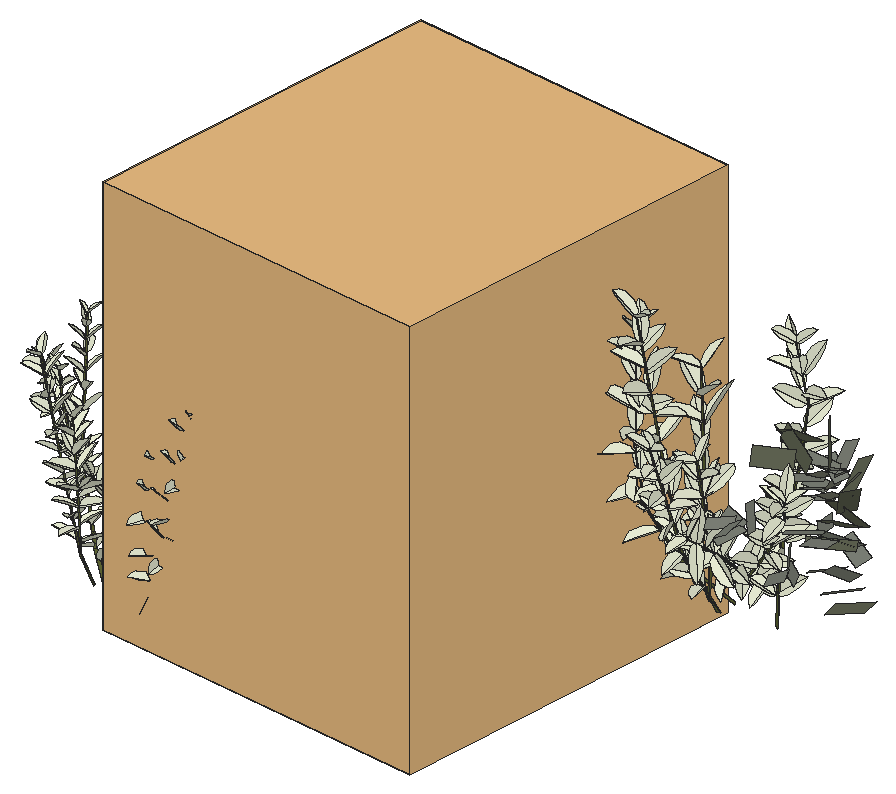
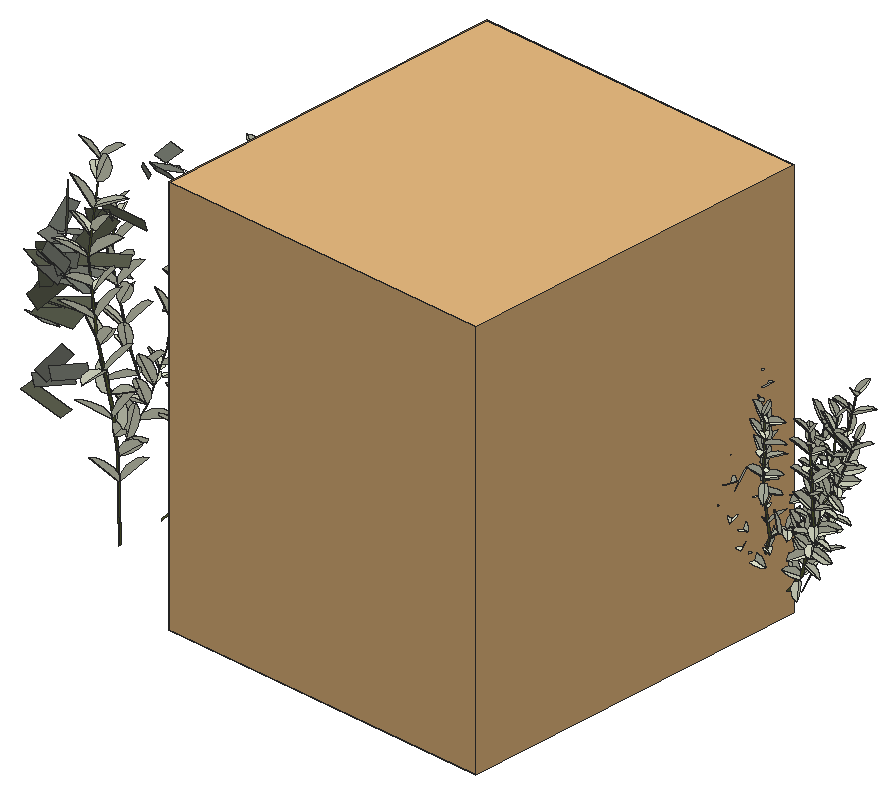
# SketchUp Ruby script. Lengths in inches.
U = 1.inch
M = Sketchup.active_model
def pt(a) = Geom::Point3d.new(a.map { |v| v * U })
def face(e, loops, mat)
  f = e.add_face(loops[0].map { |a| pt(a) })
  loops[1..].each { |l| e.add_face(l.map { |a| pt(a) }).erase! }
  f.material = f.back_material = mat if mat
  f
end
# faces: each face lists its corners as indices into pts; further lists are holes
def faces(e, pts, list, mat = nil) = list.each { |f| face(e, (f[0].is_a?(Array) ? f : [f]).map { |l| l.map { |i| pts[i] } }, mat) }
# xy, xz, yz: faces in a plane at the given z, y or x. An outline is a flat list of corners, or four numbers for a rectangle; further outlines are holes
def ring(l) = l.size == 4 ? [[l[0], l[1]], [l[2], l[1]], [l[2], l[3]], [l[0], l[3]]] : l.each_slice(2).to_a
def flat(e, list, mat, &to3) = list.each { |f| face(e, (f[0].is_a?(Array) ? f : [f]).map { |l| ring(l).map { |u, v| to3.(u, v) } }, mat) }
def xy(e, z, list, mat = nil) = flat(e, list, mat) { |x, y| [x, y, z] }
def xz(e, y, list, mat = nil) = flat(e, list, mat) { |x, z| [x, y, z] }
def yz(e, x, list, mat = nil) = flat(e, list, mat) { |y, z| [x, y, z] }
def lines(e, pts, list) = list.each { |a, b| e.add_line(pt(pts[a]), pt(pts[b])) }
# prism: a flat outline (further loops are holes) pulled along v
def prism(e, loops, v, mat = nil)
  f = face(e, loops, mat); d = Geom::Vector3d.new(v.map { |x| x * U })
  f.pushpull(f.normal.samedirection?(d) ? d.length : -d.length)
end
def box(e, o, s, mat = nil) = prism(e, [[o, [o[0] + s[0], o[1], o[2]], [o[0] + s[0], o[1] + s[1], o[2]], [o[0], o[1] + s[1], o[2]]]], [0, 0, s[2]], mat)
def at(x, y, z, deg = 0) = Geom::Transformation.translation(pt([x, y, z])) * Geom::Transformation.rotation(ORIGIN, Z_AXIS, deg.degrees)
def axes(o, x, y, z) = Geom::Transformation.new([*x, 0, *y, 0, *z, 0, *pt(o).to_a, 1])
def part(name) = M.definitions.add(name)
# library, detail: a bought-in or finely detailed component or shape, given as its bounding box
def library(name, o, s) = part(name).tap { |d| box(d.entities, o, s) }
def detail(e, o, s) = box(e.add_group.entities, o, s)
def put(e, d, t, mat = nil) = e.add_instance(d, t).tap { |i| i.material = mat if mat }
def group(e, t, mat = nil) = e.add_group.tap { |g| g.transformation = t; g.material = mat if mat }.entities
root = M.entities
M.materials.add("0ad16as01f6asdLeafVar1sfd015as60f1as6").color = [231, 235, 211]
M.materials.add("asdfasdf0165f6asdLeafVar1sfd015as60f1as6").color = [231, 235, 211]
M.materials.add("dw_stemssadfasdfa0sdf1s01d6w1").color = [90, 97, 50]
M.materials.add("viburnumblaasdfas0df1w06d").color = [98, 102, 84]
M.materials.add("viburnumbladsadfasdfad0w122").color = [125, 129, 119]
c1 = part("vdw_leaf\#2")
p = [[0,0,0],[-2.77,1.61,2.32],[-4.3125,6.1,4.5],[-3.97,13.49,6.09],[-2.47,18.57,6.3],[-0.2,22.73,5.75],
  [2.54,19.66,6.85],[4.3,15.93,7.09],[5.03,7.6,5.43],[3.32,1.76,2.74]]
faces(c1.entities,p,[[0,1,2,3,4,5],[0,5,6,7,8,9]],"asdfasdf0165f6asdLeafVar1sfd015as60f1as6")
c2 = part("dg_branch_1\#2")
p = [[46.12,1.57,35.62],[46,5.42,35.41],[0.14,1.79,0.05],[0.26,-2.0625,0.27],[74.05,2.99,75.8],[74.11,5.28,75.58],
  [103.46,0.47,94.74],[104.03,2.92,94.84],[81.14,16.92,120.46],[81.2,18.78,120.24],[130.47,-5.6875,130.27],[130.58,-3.66,129.85],
  [80.82,34.4375,191.22],[80.64,35.93,190.9],[148.49,-14.56,203.24],[148.9,-12.8125,203.11],[81.08,37.95,226.93],[81.4,39.1,227.03],
  [157.45,-18.19,250.77],[157.7,-17.01,250.41]]
faces(c2.entities,p,[[0,1,2,3],[4,0,1],[4,1,5],[6,4,5],[6,5,7],[8,4,5],[8,5,9],[10,6,7],
  [10,7,11],[12,8,9],[12,9,13],[14,10,11],[14,11,15],[16,12,13],[16,13,17],[18,14,15],
  [18,15,19]],"dw_stemssadfasdfa0sdf1s01d6w1")
c3 = part("vdw_branch1\#3")
put(c3.entities,c1,axes([120.69,-2.42,117.31],[1.12221,-0.24063,-0.65809],[0.19207,1.24776,-0.12871],[0.65778,0.01392,1.11658]))
put(c3.entities,c1,axes([81,38.9,226.05],[0.7888,-0.58155,0],[0.48308,0.65523,0.47],[-0.28484,-0.38635,0.83138]))
put(c3.entities,c1,axes([78.08,12.69,106.05],[-1.43826,-0.02353,-0.03177],[0.0088,-1.31777,0.57755],[-0.03854,0.57714,1.31741]))
put(c3.entities,c1,axes([130.18,-4.73,130.41],[-0.38031,-1.29044,-0.11242],[1.20662,-0.31032,-0.51987],[0.47109,-0.24694,1.24081]))
put(c3.entities,c1,axes([157.08,-17.89,249.93],[-0.91355,0.40674,0],[-0.37496,-0.84216,0.38752],[0.15762,0.35401,0.92186]))
put(c3.entities,c1,axes([90.64,3.03,86.49],[0.32514,-0.85045,-0.99675],[0.69523,0.98247,-0.61148],[1.11061,-0.36604,0.67459]))
put(c3.entities,c1,axes([80.15,28.42,160.95],[-0.16039,0.95636,-1.06292],[-1.41646,0.03966,0.24943],[0.19509,1.07422,0.93709]))
put(c3.entities,c1,axes([126.74,-5.45,129.22],[-0.59819,0.96152,-0.6841],[-0.85772,0.12575,0.92675],[0.75427,0.88089,0.57856]))
put(c3.entities,c1,axes([133.22,-6.12,150.66],[-0.93823,0.76985,0.59124],[-0.47726,-1.08188,0.65135],[0.84525,0.24366,1.02405]))
put(c3.entities,c1,axes([80.43,22.89,141.32],[-1.42571,-0.19312,0.01373],[0.18338,-1.31425,0.5561],[-0.0621,0.5528,1.32692]))
put(c3.entities,c1,axes([33.14,0.88,26.42],[-0.13338,1.31536,0.04876],[-1.04528,-0.13221,0.7073],[0.72315,0.03348,1.07497]))
put(c3.entities,c1,axes([152.63,-15.08,221.76],[-1.28188,0.41945,0.0579],[-0.3638,-1.18547,0.53367],[0.21665,0.49113,1.23869]))
put(c3.entities,c1,axes([80.05,28.28,160.33],[-0.46732,-1.26661,0.40679],[1.27397,-0.40257,0.21004],[-0.07408,0.44645,1.30501]))
put(c3.entities,c1,axes([153.95,-14.8,235.875],[0.39005,1.07743,0.20605],[-0.96443,0.25296,0.50293],[0.42961,-0.3464,0.99807]))
put(c3.entities,c1,axes([80.2,24.22,141.74],[1.33062,-0.46576,0.02628],[0.44746,1.2746,-0.06608],[-0.00197,0.0722,1.37936]))
put(c3.entities,c1,axes([145.48,-12.5,188.92],[-1.32952,0.16983,0.16138],[-0.09299,-1.2361,0.53471],[0.21503,0.51548,1.22904]))
put(c3.entities,c1,axes([139.64,-9.18,171.24],[0.05682,1.30088,0.23414],[-1.13176,-0.05343,0.57151],[0.58357,-0.22963,1.13417]))
put(c3.entities,c1,axes([70.95,4.35,71.98],[-1.1081,-0.41873,0.64752],[0.33675,-1.28259,-0.25313],[0.6937,-0.04625,1.15721]))
put(c3.entities,c1,axes([59.85,4.55,56.17],[-0.26797,1.24526,0.35754],[-0.9369,-0.41634,0.74783],[0.83377,-0.10389,0.98674]))
put(c3.entities,c1,axes([33.11,3.36,25.66],[-0.57817,-1.07968,-0.5679],[1.11554,-0.21356,-0.7297],[0.49375,-0.78178,0.98363]))
put(c3.entities,c2,at(-0.21,0.34,-0.17),"dw_stemssadfasdfa0sdf1s01d6w1")
put(c3.entities,c1,axes([80.91,19.01,122.53],[-0.84258,1.13222,-0.27981],[-1.15093,-0.75138,0.42537],[0.18861,0.47293,1.3457]))
put(c3.entities,c1,axes([119.8,-1.22,114.1],[-1.3235,-0.25012,0.09101],[0.25933,-1.31572,0.15537],[0.05991,0.1698,1.33794]))
put(c3.entities,c1,axes([46.29,5.1,38.04],[0.98937,0.73827,-0.47585],[-0.72359,1.03721,0.10473],[0.44068,0.18581,1.20453]))
put(c3.entities,c1,axes([81.1875,33.03,184.45],[1.33883,0.26986,0.35053],[-0.09581,1.22087,-0.57399],[-0.42216,0.53228,1.20262]))
put(c3.entities,c1,axes([80.16,36.28,206.98],[-0.83993,0.85737,-0.6234],[-1.05964,-0.65701,0.5241],[0.02941,0.81391,1.07976]))
put(c3.entities,c1,axes([154.86,-16.15,234.87],[0.02509,-1.15302,-0.28506],[1.1487,-0.04894,0.29908],[-0.30202,-0.28195,1.11384]))
put(c3.entities,c1,axes([108.77,-0.33,101.14],[-0.47691,-1.03266,-0.72709],[1.25395,-0.29455,-0.40416],[0.15052,-0.81814,1.06325]))
put(c3.entities,c1,axes([89.79,3.01,85.87],[-0.61344,0.75518,0.8965],[-0.17758,-1.01824,0.73622],[1.13385,0.22574,0.58569]))
put(c3.entities,c1,axes([81.56,20.31,123.29],[0.37259,-1.3435,0.21057],[1.29385,0.32364,-0.22445],[0.16906,0.25791,1.34638]))
put(c3.entities,c1,axes([46.45,1.82,36.74],[-0.77883,0.29892,1.0614],[0.19124,-1.24314,0.49044],[1.08598,0.43329,0.67484]))
put(c3.entities,c1,axes([71.37,4.02,72.32],[0.72905,0.81546,-0.74421],[-0.66805,0.98958,0.42988],[0.8391,0.14186,0.97745]))
put(c3.entities,c1,axes([136.59,-5.88,150.53],[0.85845,-0.99897,-0.12437],[0.96526,0.81273,0.13453],[-0.02572,-0.18182,1.28292]))
put(c3.entities,c1,axes([80.375,38.8,225.86],[-0.25178,0.96778,0],[-0.89216,-0.23211,0.38752],[0.37503,0.09757,0.92186]))
put(c3.entities,c1,axes([74.43,7.99,85.38],[-1.05703,0.91669,-0.33543],[-0.95806,-0.87958,0.61531],[0.18697,0.6754,1.25659]))
put(c3.entities,c1,axes([76.57,9.74,89.32],[0.63146,-1.21538,0.33508],[1.18148,0.49387,-0.43517],[0.26321,0.48577,1.26593]))
put(c3.entities,c1,axes([81.6875,36.97,207.4],[0.09422,-1.04424,0.38486],[1.01646,0.1939,0.27727],[-0.33299,0.33382,0.98727]))
put(c3.entities,c1,axes([157.29,-17.17,249.98],[0.50586,-0.50586,0],[0.38853,0.38853,0.41105],[-0.29684,-0.29684,0.56115]))
put(c3.entities,c1,axes([79.92,15.8,106.09],[1.03917,-0.29343,-0.90675],[-0.14587,1.22131,-0.5624],[0.92163,0.5191,0.88824]))
put(c3.entities,c1,axes([61.95,3.88,56.26],[0.41243,-1.28546,0],[1.17466,0.37688,-0.54831],[0.5221,0.16751,1.23363]))
put(c3.entities,c1,axes([151.99,-14.79,208.15],[-0.48571,-1.21723,-0.32393],[1.25386,-0.50033,0],[-0.12005,-0.30087,1.31056]))
put(c3.entities,c1,axes([108.44,0.62,102.22],[0.82183,0.96078,0.38967],[-0.62327,0.08618,1.10203],[0.79141,-0.88661,0.51693]))
put(c3.entities,c1,axes([145.6,-10.56,188.62],[1.03241,-0.02554,-0.82693],[0.3944,1.11584,0.45794],[0.70325,-0.61672,0.89706]))
put(c3.entities,c1,axes([78.59,32.3,183.89],[-1.12675,-0.42036,0.43987],[0.5899,-0.98149,0.57312],[0.14901,0.70693,1.05726]))
put(c3.entities,c1,axes([152.08,-13.42,223.37],[0.79993,-0.44251,-0.69938],[0.68456,0.82615,0.26026],[0.41048,-0.60953,0.85515]))
put(c3.entities,c1,axes([140.71,-8.74,170.55],[0.41903,-1.24177,-0.32393],[1.26224,0.33728,0.33986],[-0.23168,-0.40836,1.26573]))
put(c3.entities,c1,axes([149.25,-12.53,205.78],[1.24456,0.38285,0.23414],[-0.42999,1.04826,0.57151],[-0.02056,-0.62679,1.13417]))
c4 = part("vdw_leaf\#3")
p = [[0,0,0],[-2.77,1.61,2.32],[-4.3125,6.1,4.5],[-3.97,13.49,6.09],[-2.47,18.57,6.3],[-0.2,22.73,5.75],
  [2.54,19.66,6.85],[4.3,15.93,7.09],[5.03,7.6,5.43],[3.32,1.76,2.74]]
faces(c4.entities,p,[[0,1,2,3,4,5],[0,5,6,7,8,9]],"asdfasdf0165f6asdLeafVar1sfd015as60f1as6")
c5 = part("dw_brancj_2\#2")
p = [[9.7,-0.22,29.95],[0.23,-1.96,0.34],[-0.05,1.51,0.11],[9.65,1.51,29.46],[18.64,-8.75,84.43],[18.96,-6.63,84.625],
  [1.53,6.02,63.68],[1.42,8.18,63.25],[-10.58,8.77,161.17],[-10.41,9.98,160.68],[26.34,-9.37,211.72],[26.57,-8.28,211.23]]
faces(c5.entities,p,[[0,1,2],[0,2,3],[4,0,3],[4,3,5],[6,0,3],[6,3,7],[8,6,7],[8,7,9],
  [10,4,5],[10,5,11]],"dw_stemssadfasdfa0sdf1s01d6w1")
c6 = part("vdw_branch2\#3")
put(c6.entities,c4,axes([19.53,-5.9,102.42],[1.12377,-0.50004,0],[0.46097,1.03596,0.47664],[-0.19377,-0.43548,1.13389]))
put(c6.entities,c4,axes([-5.89,6.52,109.44],[-1.07209,0.83679,0],[-0.77141,-0.98832,0.52702],[0.32427,0.41545,1.25373]))
put(c6.entities,c4,axes([-0.44,8.23,75.28],[0.88709,-0.9947,0],[0.92159,0.82189,0.33087],[-0.25219,-0.22491,1.26111]))
put(c6.entities,c4,axes([24.71,-8.97,190.81],[-0.82641,0.91101,0],[-0.83983,-0.76184,0.47664],[0.35303,0.32025,1.13389]))
put(c6.entities,c4,axes([-2.29,8.24,91.35],[1.24603,-0.47303,0],[0.43826,1.15445,0.33087],[-0.11993,-0.31592,1.26111]))
put(c6.entities,c4,axes([12.26,-3.11,37.92],[-0.64625,1.02205,0.22511],[-1.04383,-0.61044,-0.22511],[-0.07533,-0.30931,1.18809]))
put(c6.entities,c4,axes([26.17,-9.17,210.27],[-0.99452,-0.10453,0],[0.09636,-0.91681,0.38752],[-0.04051,0.38539,0.92186]))
put(c6.entities,c4,axes([-6.07,9.4,125.35],[-0.90214,-0.98107,0],[0.90896,-0.83583,0.33087],[-0.24874,0.22873,1.26111]))
put(c6.entities,c4,axes([-4.13,7.29,110.58],[0.44715,-1.078,0.64369],[1.05816,0.63649,0.33087],[-0.58725,0.40856,1.09216]))
put(c6.entities,c4,axes([23.91,-8.22,171.96],[0.62307,0.85009,-0.63406],[-0.71531,0.8798,0.47664],[0.78296,0.12729,0.94004]))
put(c6.entities,c5,at(-0.09,0.18,-0.25),"dw_stemssadfasdfa0sdf1s01d6w1")
put(c6.entities,c4,axes([23.34,-9.65,156.59],[-0.31364,-1.00782,0.58216],[1.10369,-0.17062,0.29925],[-0.17137,0.6239,0.98776]))
put(c6.entities,c4,axes([15.03,-3.37,58.83],[-1.05425,-0.00194,0.58442],[-0.14303,-1.11707,-0.26172],[0.55355,-0.3046,0.99755]))
put(c6.entities,c4,axes([-11.625,9.46,160.37],[0.36812,0.92978,0],[-0.85713,0.33936,0.38752],[0.3603,-0.14265,0.92186]))
put(c6.entities,c4,axes([21.32,-8.53,138.72],[1.21379,0.19904,0],[-0.19904,1.21379,0],[0,0,1.23]))
put(c6.entities,c4,axes([22.54,-9.2,141.43],[-1.02887,0.17955,0.60182],[-0.23387,-1.13057,-0.06253],[0.56696,-0.17376,1.02111]))
put(c6.entities,c4,axes([23.9,-8.82,173.84],[-1.14567,-0.37474,0],[0.35918,-1.0981,0.04438],[-0.01409,0.04308,1.17993]))
put(c6.entities,c4,axes([-7.84,8.92,143.59],[-1.26971,0.40522,0],[-0.37543,-1.17638,0.33087],[0.10274,0.32192,1.26111]))
put(c6.entities,c4,axes([19.77,-8.01,85.98],[-0.32405,-1.14591,0.18674],[1.10278,-0.32969,-0.10948],[0.15845,0.14442,1.16117]))
put(c6.entities,c4,axes([-0.62,5.76,76.34],[-0.08879,1.17576,-0.67771],[-1.34525,-0.16582,-0.11144],[-0.17897,0.66309,1.17383]))
put(c6.entities,c4,axes([20.49,-8.22,121.07],[0.39924,-0.78471,-0.8233],[1.08735,0.33121,0.2116],[0.09035,-0.83005,0.83495]))
put(c6.entities,c4,axes([15.15,-3.72,62.9],[1.16251,0.40128,-0.0211],[-0.39924,1.16074,0.07874],[0.0456,-0.06757,1.2273]))
put(c6.entities,c4,axes([20.72,-8.08,120.26],[-0.03693,1.2277,-0.06551],[-1.22944,-0.03698,0],[-0.00197,0.06548,1.22825]))
put(c6.entities,c4,axes([22.58,-8.36,155.57],[-0.56247,1.09386,0],[-1.00839,-0.51852,0.47664],[0.42389,0.21796,1.13389]))
put(c6.entities,c4,axes([3.97,3.13,57.96],[-1.09459,0.76041,0],[-0.72262,-1.0402,-0.1735],[-0.10109,-0.14552,1.29352]))
put(c6.entities,c4,axes([-10.8,9.06,160.75],[-0.66334,-0.72138,0],[0.66835,-0.61458,0.24329],[-0.1829,0.16818,0.92729]))
put(c6.entities,c4,axes([19.06,-9.3125,103.96],[-1.01345,0.25553,-0.60051],[-0.2265,-1.12952,-0.09839],[-0.59598,0.03076,1.01889]))
put(c6.entities,c4,axes([18.07,-6.2,81.7],[-0.56247,1.09386,0],[-1.00839,-0.51852,0.47664],[0.42389,0.21796,1.13389]))
put(c6.entities,c4,axes([12.95,-0.39,43.31],[0.13044,-1.19832,0],[1.11025,0.12085,0.29925],[-0.30382,-0.03307,1.14057]))
put(c6.entities,c4,axes([2.28,8.28,56.18],[1.32413,-0.31027,0],[0.30923,1.31968,-0.11144],[0.02542,0.1085,1.35543]))
put(c6.entities,c4,axes([-7.55,9.96,143.07],[1.34251,-0.21744,0],[0.20045,1.23761,0.52702],[-0.08426,-0.52024,1.25373]))
put(c6.entities,c4,axes([26.15,-8.25,210.66],[0.94661,-0.25364,0],[0.235,0.87703,0.24329],[-0.06431,-0.24,0.92729]))
put(c6.entities,c4,axes([-6.48,11.37,125.16],[0.64635,1.10315,0.46356],[-1.16569,0.46153,0.52702],[0.27017,-0.6478,1.16488]))
put(c6.entities,c4,axes([25.74,-8.35,191.28],[0.13044,-1.19832,0],[1.11025,0.12085,0.29925],[-0.30382,-0.03307,1.14057]))
put(c6.entities,c4,axes([-5.125,7.47,91.6],[-1.10024,0.63688,0.48318],[-0.78682,-1.00808,-0.46292],[0.14137,-0.65404,1.184]))
c7 = part("vdw_leaf\#1")
p = [[0,0,0],[-2.77,1.61,2.32],[-4.3125,6.1,4.5],[-3.97,13.49,6.09],[-2.47,18.57,6.3],[-0.2,22.73,5.75],
  [2.54,19.66,6.85],[4.3,15.93,7.09],[5.03,7.6,5.43],[3.32,1.76,2.74]]
faces(c7.entities,p,[[0,1,2,3,4,5],[0,5,6,7,8,9]],"0ad16as01f6asdLeafVar1sfd015as60f1as6")
c8 = part("dw_branch_3\#2")
p = [[-10.06,-1.6,62.9],[-0.2,1.54,-0.01],[-10.43,1.54,62.72],[0.18,-1.6,0.17],[-23.75,-21.66,88.91],[-25.7,-20.3,89.55],
  [13.4,11.62,104.56],[13.33,13.52,104.47],[-49.25,-41.87,130.3125],[-50.33,-40.21,130.71],[-4.97,21.13,143.98],[35.61,27.99,178.64],
  [-5.09,23.64,143.96],[35.32,29.14,178.46],[-67.7,-55.38,181.06],[-68.34,-54.45,181.62],[-22.8125,33.9,200.59],[-22.94,35.79,200.41],
  [56.61,36.78,229.75],[56.29,38.09,229.57],[-70.63,-67.46,248.85],[-70.72,-66.33,249.5],[-25.05,43.32,240.75],[-24.98,44.26,240.57]]
faces(c8.entities,p,[[0,1,2],[0,3,1],[4,2,5],[4,0,2],[6,0,2],[6,2,7],[8,4,5],[8,5,9],
  [10,6,7],[11,6,7],[10,7,12],[11,7,13],[14,8,9],[14,9,15],[16,10,12],[16,12,17],
  [18,11,13],[18,13,19],[20,14,15],[20,15,21],[22,16,17],[22,17,23]],"dw_stemssadfasdfa0sdf1s01d6w1")
c9 = part("dw_branch3\#2")
put(c9.entities,c7,axes([-70.33,-63.58,233.32],[-1.00752,0.412,0.78596],[-0.24851,-1.22189,0.32195],[0.83141,0.09817,1.01433]))
put(c9.entities,c7,axes([-66.93,-54.91,182.82],[-0.84976,-0.98359,0.33619],[0.99572,-0.74889,0.32577],[-0.05223,0.46521,1.22907]))
put(c9.entities,c7,axes([-46.12,-39.49,126.35],[1.23843,0.5364,0.23552],[-0.56438,0.94474,0.81599],[0.15707,-0.83465,1.07498]))
put(c9.entities,c7,axes([13.0625,13.13,104.77],[-1.01271,0.69982,-0.26884],[-0.74268,-0.99813,0.19939],[-0.10222,0.31872,1.21473]))
put(c9.entities,c7,axes([-18.87,30.42,186.42],[0.36309,1.06515,-0.56675],[-1.14134,0.49515,0.19939],[0.39128,0.45593,1.10754]))
put(c9.entities,c7,axes([-3.2,4.15,75.77],[-1.04153,0.55414,0.44243],[-0.23365,-1.01045,0.71554],[0.6695,0.50943,0.93801]))
put(c9.entities,c7,axes([23.2,19.41,136.3],[-0.65687,-1.11295,-0.05714],[1.05857,-0.61429,-0.20411],[0.15163,-0.1536,1.24868]))
put(c9.entities,c7,axes([-25.57,35.48,201.32],[-0.64726,0.62827,0.87973],[-0.71635,-1.0172,0.19939],[0.80962,-0.39773,0.87973]))
put(c9.entities,c7,axes([-36.37,-32.14,110.35],[-0.80747,1.09962,0.12544],[-0.83333,-0.50188,-0.96467],[-0.72833,-0.64487,0.96467]))
put(c9.entities,c7,axes([-9.89,26.72,156.79],[0.45529,1.02969,0.56572],[-1.16919,0.33753,0.32662],[0.11537,-0.64297,1.07744]))
put(c9.entities,c7,axes([-26.57,46.1,241.0625],[0.00015,0.80921,0.22536],[-0.83985,0.00446,-0.01542],[-0.01605,-0.22532,0.80906]))
put(c9.entities,c7,axes([-9.2,-2.58,61.06],[-1.10001,-0.40312,0.39014],[0.40883,-1.1116,0.00411],[0.35732,0.13566,1.14763]))
put(c9.entities,c7,axes([-69.91,-63.11,233.93],[1.36249,-0.1432,0],[0.13201,1.25603,0.5309],[-0.05549,-0.52799,1.26295]))
put(c9.entities,c7,axes([32.2,25.46,166.13],[0.06878,-1.29051,-0.05714],[1.22165,0.07415,-0.20411],[0.2113,-0.04403,1.24868]))
put(c9.entities,c7,axes([-5.68,-0.66,44.43],[-0.48448,-1.12287,0.17078],[0.98138,-0.33653,0.57135],[-0.48308,0.36756,1.04626]))
put(c9.entities,c7,axes([43.45,32.81,198.64],[0.5408,1.19584,0.14106],[-0.94242,0.32409,0.86557],[0.74952,-0.45533,0.98656]))
put(c9.entities,c7,axes([12.52,14.14,104.98],[1.02694,0.54888,0.41092],[-0.53566,1.05407,-0.06927],[-0.38969,-0.12321,1.13846]))
put(c9.entities,c7,axes([44.55,32.375,198.73],[-0.65687,-1.11295,-0.05714],[1.05857,-0.61429,-0.20411],[0.15163,-0.1536,1.24868]))
put(c9.entities,c7,axes([-5.67,21.17,141.44],[-1.10726,0.43603,-0.32953],[-0.49537,-1.03435,0.29588],[-0.17521,0.40597,1.12589]))
put(c9.entities,c7,axes([55.69,37.84,229.48],[0.18984,0.96334,0.18958],[-0.71996,0.0053,0.69399],[0.66755,-0.26823,0.69457]))
put(c9.entities,c7,axes([-21.52,36.85,205.2],[0.72606,-0.98817,0.14519],[0.94364,0.7084,0.10251],[-0.16885,0.05176,1.19664]))
put(c9.entities,c7,axes([-68.51,-56.35,196.07],[1.16319,0.72381,0],[-0.66725,1.0723,0.5309],[0.28049,-0.45075,1.26295]))
put(c9.entities,c8,at(0.01,-0.09,-0.02),"dw_stemssadfasdfa0sdf1s01d6w1")
put(c9.entities,c7,axes([-2.49,5.18,75.91],[0.78614,-0.90346,-0.30078],[0.86953,0.79562,-0.11715],[0.28546,-0.14014,1.16705]))
put(c9.entities,c7,axes([-23.125,-16.22,82.25],[0.32175,1.32576,0.12544],[-1.33153,0.31835,0.05068],[0.01989,-0.13382,1.3633]))
put(c9.entities,c7,axes([-23.75,41.99,230.3],[0.85958,-0.87451,0.14519],[0.66531,0.75721,0.62192],[-0.54076,-0.36226,1.01955]))
put(c9.entities,c7,axes([27.07,22.48,149.34],[0.92952,-0.64745,-0.62467],[0.50188,1.074,-0.36637],[0.71693,0.02135,1.04468]))
put(c9.entities,c7,axes([17.66,16.25,119.93],[-0.91649,0.83891,-0.3601],[-0.87434,-0.77966,0.40896],[0.0492,0.54447,1.14321]))
put(c9.entities,c7,axes([-68.37,-54.54,181.63],[0.32047,1.28399,0.35434],[-1.33153,0.31835,0.05068],[-0.03484,-0.35624,1.32241]))
put(c9.entities,c7,axes([-28.98,-27.1,96.48],[-0.8814,-0.35966,-0.98523],[0.75246,-1.11336,-0.26672],[-0.73065,-0.71272,0.91382]))
put(c9.entities,c7,axes([-15.23,28.43,172.72],[-1.21149,0.11898,0.32517],[-0.09739,-1.25259,0.09551],[0.33228,0.0667,1.21356]))
put(c9.entities,c7,axes([-17.5625,31.23,186.85],[-0.49275,-1.12287,0.14519],[0.95014,-0.33653,0.62192],[-0.53717,0.36756,1.01955]))
put(c9.entities,c7,axes([26.7,21.22,149.39],[-1.00104,0.22334,0.83093],[0.36894,-1.0402,0.72406],[0.77731,0.78134,0.72643]))
put(c9.entities,c7,axes([-31.125,-24.87,97.38],[0.75482,-0.86936,0.69068],[-0.00159,0.80023,1.00899],[-1.08766,-0.58016,0.45842]))
put(c9.entities,c7,axes([-71.21,-66.73,248.67],[0.25207,0.96771,0],[-0.8921,0.23237,0.38752],[0.375,-0.09768,0.92186]))
put(c9.entities,c7,axes([-24.11,41.05,229.55],[-1.11612,0.51924,-0.26884],[-0.56394,-1.10897,0.19939],[-0.15444,0.29694,1.21473]))
put(c9.entities,c7,axes([6.75,8.37,91.63],[-0.33418,-1.12287,0.39014],[1.13558,-0.33653,0.00411],[0.10478,0.36756,1.14763]))
put(c9.entities,c7,axes([-26,45.89,241.63],[-0.26986,-0.70824,-0.32129],[0.56818,-0.39091,0.38449],[-0.49365,-0.09775,0.63011]))
put(c9.entities,c7,axes([3.74,17.32,124.35],[0.22441,1.22913,-0.16274],[-1.07812,0.11178,-0.64246],[-0.61228,0.25367,1.07162]))
put(c9.entities,c7,axes([-5.44,22.27,140.88],[1.2203,0.00475,0.31374],[-0.097,1.20386,0.35905],[-0.29841,-0.37189,1.1663]))
put(c9.entities,c7,axes([-13.79,29.35,173.31],[0.83169,-0.90108,0.14519],[0.68877,0.73594,0.62192],[-0.55187,-0.34509,1.01955]))
put(c9.entities,c7,axes([-16.92,-7.26,72.98],[1.30647,0.30378,-0.27886],[0.07026,0.74892,1.14503],[0.40633,-1.10623,0.69861]))
put(c9.entities,c7,axes([4.8,17.55,125.22],[-0.25598,-1.17842,0.26559],[1.01553,-0.08455,0.60363],[-0.56975,0.35087,1.00767]))
put(c9.entities,c7,axes([5.3125,8.35,91.45],[0.00638,1.22913,-0.27714],[-1.16413,0.11178,0.46895],[0.48205,0.25367,1.13617]))
put(c9.entities,c7,axes([38.12,30.57,183.07],[1.12534,0.26182,-0.63833],[-0.46674,1.18829,-0.33545],[0.5081,0.51169,1.10563]))
put(c9.entities,c7,axes([-70.41,-60.38,214.47],[-0.41425,1.30587,0],[-1.20383,-0.38188,0.5309],[0.50605,0.16053,1.26295]))
put(c9.entities,c7,axes([37.03,28.75,180.67],[-1.12533,0.00102,-0.63799],[-0.00113,-1.2408,0],[-0.62497,0.00057,1.10237]))
put(c9.entities,c7,axes([30.71,25.35,165.96],[-0.1364,1.29314,0.22715],[-1.08768,-0.23921,0.70862],[0.73536,-0.11394,1.09026]))
put(c9.entities,c7,axes([-38.05,-30.84,110.67],[-0.31533,-1.27379,-0.2839],[1.018,-0.40311,0.67794],[-0.74394,-0.05723,1.08307]))
put(c9.entities,c7,axes([50.11,34.45,213.36],[-1.05669,0.74401,-0.05714],[-0.616,-0.82138,0.69675],[0.37221,0.60904,1.04705]))
put(c9.entities,c7,axes([-65.32,-58.78,200.07],[-1.14597,-0.19668,-0.6713],[0.21784,-1.26924,0],[-0.64812,-0.11124,1.139]))
put(c9.entities,c7,axes([-53.2,-43.37,143.59],[-0.72817,-1.09167,-0.2839],[0.82127,-0.72411,0.67794],[-0.71934,0.19815,1.08307]))
put(c9.entities,c7,axes([-61.1,-50.25,163.67],[-0.52887,1.19686,-0.30066],[-1.10762,-0.57104,-0.32484],[-0.42634,0.12264,1.23812]))
put(c9.entities,c7,axes([-54.12,-42.96,142.67],[0.32175,1.32576,0.12544],[-1.33153,0.31835,0.05068],[0.01989,-0.13382,1.3633]))
put(c9.entities,c7,axes([22.03,20.08,132.3],[1.17066,0.5058,-0.34078],[-0.35758,1.16671,0.50333],[0.49407,-0.35407,1.17172]))
put(c9.entities,c7,axes([-8.59,26.04,158.21],[-0.49275,-1.12287,0.14519],[0.95014,-0.33653,0.62192],[-0.53717,0.36756,1.01955]))
put(c9.entities,c7,axes([49.92,34.03,213.7],[1.24742,-0.35176,0.25024],[0.42127,1.159,-0.4708],[-0.09426,0.52477,1.20753]))
put(c9.entities,c7,axes([-70.34,-67.02,249.05],[-0.57048,-0.79684,0],[0.73827,-0.52855,0.24329],[-0.20203,0.14464,0.92729]))
put(c9.entities,c7,axes([56.04,36.81,228.63],[0.33451,-0.90845,-0.15237],[0.87636,0.33365,-0.06538],[0.11487,-0.11636,0.94597]))
put(c9.entities,c7,axes([-69.93,-60.58,214.88],[-0.45293,-0.99272,-0.78227],[1.14635,-0.58199,0.07483],[-0.40282,-0.65636,1.06615]))
put(c9.entities,c7,axes([-16.77,-8.59,72.7],[-1.22785,0.11509,0.53076],[-0.24879,-1.22495,-0.30991],[0.46742,-0.38989,1.16587]))
put(c9.entities,c7,axes([18.29,17.18,119.24],[1.19981,-0.45946,0.3029],[0.40159,1.22775,0.27158],[-0.37626,-0.1547,1.25575]))
put(c9.entities,c7,axes([-6.73,-0.68,43.74],[0.05346,1.22913,-0.27201],[-1.22696,0.11178,0.26396],[0.28163,0.25367,1.20164]))
put(c9.entities,c7,axes([-58.57,-48.42,160.98],[0.43385,-1.23789,0.39533],[1.04879,0.57965,0.66404],[-0.76727,0.09236,1.13122]))
put(c9.entities,c7,axes([-23.4,38.49,215.38],[0.06762,1.22913,-0.26884],[-1.23909,0.11178,0.19939],[0.21835,0.25367,1.21473]))
put(c9.entities,c7,axes([-22.21,-16.62,83.17],[-0.72817,-1.09167,-0.2839],[0.82127,-0.72411,0.67794],[-0.71934,0.19815,1.08307]))
put(c9.entities,c7,axes([-45.7,-40.77,126.53],[-1.33715,-0.0713,-0.0976],[0.07167,-1.28508,-0.04314],[-0.09306,-0.0492,1.31098]))
put(c9.entities,c7,axes([-22.39,38.51,216.12],[-0.49275,-1.12287,0.14519],[0.95014,-0.33653,0.62192],[-0.53717,0.36756,1.01955]))
c10 = library("Narrowleaf plant",[-0.44,-0.75,-1.28],[7.48,8.05,9.01])
c11 = part("Component\#314")
p = [[0.14,0,0],[2.58,0.05,0.25],[2.44,5.11,2.64],[0,5.05,2.39]]
faces(c11.entities,p,[[0,1,2,3]],"viburnumblaasdfas0df1w06d")
c12 = part("viburnumblad1\#2")
put(c12.entities,c11,axes([-37.25,6.23,19.31],[75.98784,0,0],[0,65.50676,0],[0,0,75.98784]))
c13 = part("Component\#315")
p = [[0.25,0,0],[2.05,0.01,0.35],[1.81,4.2,1.66],[0,4.19,1.3125]]
faces(c13.entities,p,[[0,1,2,3]],"viburnumbladsadfasdfad0w122")
c14 = part("viburnumblad2")
put(c14.entities,c13,axes([-19.23,-4.49,-32.18],[83.35428,0,0],[0,79.38502,0],[0,0,83.35428]))
put(root,c3,axes([1134.98,250.39,-3.7],[-0.07583,0.05409,0],[-0.05409,-0.07583,0],[0,0,0.11461]))
put(root,c6,axes([1132.82,250.44,-2.94],[-0.10632,-0.02382,-0.02533],[0.02424,-0.1082,0],[-0.02009,-0.0045,0.13407]))
put(root,c9,axes([1136.93,253.08,-1.4],[0.06434,-0.05829,0.02833],[0.05722,0.06809,0.01535],[-0.02555,0.00573,0.10572]))
put(root,c6,axes([1137.5,251.76,-4.3],[0.00659,0.0958,-0.06822],[-0.11062,0.0076,0],[0.0038,0.05531,0.11816]))
put(root,c6,axes([1140.29,249.17,-4.8],[0.01852,0.08442,-0.0614],[-0.09748,0.02138,0],[0.01069,0.04874,0.10635]))
put(root,c6,axes([1140.9,248.71,-2.94],[0.10716,0.01972,-0.02533],[-0.02007,0.10905,0],[0.02025,0.00373,0.13407]))
put(root,c3,axes([1139.39,249.66,-3.7],[0.07973,0.03352,0],[-0.03352,0.07973,0],[0,0,0.10642]))
put(root,c10,axes([1138.49,253.56,1.02],[6.41217,-0.58355,0],[0.58355,6.41217,0],[0,0,6.43866]))
put(root,c3,axes([1195.78,287.68,0.51],[-0.11019,-0.08184,0],[0.08184,-0.11019,0],[0,0,0.16889]))
put(root,c6,axes([1194.73,284.69,1.63],[-0.01475,-0.15988,-0.03733],[0.16271,-0.01501,0],[-0.00279,-0.03021,0.19757]))
put(root,c6,axes([1196.05,284.4,0.89],[0.0254,-0.1143,-0.07152],[0.12761,0.02836,0],[0.01261,-0.05674,0.14408]))
put(root,c9,axes([1199.36,290.81,-2.75],[-0.08978,-0.1003,-0.04713],[0.10044,-0.06083,-0.0937],[0.03793,-0.07633,0.13659]))
put(root,c12,axes([1212.32,281.99,26.61],[-0.00628,0.01217,-0.00276],[-0.013,-0.00799,-0.00559],[-0.00514,0.00045,0.01101]))
put(root,c12,axes([1211.61,283.65,28.55],[-0.01179,-0.00065,-0.00527],[-0.00088,-0.01435,0.00336],[-0.0049,0.00375,0.00968]))
put(root,c12,axes([1213.9375,276.13,29.375],[-0.00239,0.00794,0.01052],[-0.01424,0.00397,-0.00606],[-0.00563,-0.01073,0.00596]))
put(root,c14,axes([1213.11,281.88,25.32],[-0.00442,0.0106,-0.0025],[-0.00963,-0.00512,-0.00451],[-0.00488,0.00074,0.00902]))
put(root,c14,axes([1213.22,281.79,23.85],[0.00321,0.01115,0.00217],[-0.01022,0.00386,-0.00469],[-0.00482,-0.00036,0.00904]))
put(root,c12,axes([1214.09,278.2,27.96],[0.00666,0.0005,0.01169],[-0.01037,0.01092,0.00488],[-0.00799,-0.01005,0.00435]))
put(root,c14,axes([1213.93,285.08,13.09],[-0.00591,0.00596,-0.00904],[-0.00601,-0.0106,-0.00307],[-0.00924,0.00313,0.00728]))
put(root,c14,axes([1214.63,281.79,23.36],[-0.00355,0.00962,-0.00319],[-0.00963,-0.00512,-0.00451],[-0.00533,0.00188,0.0087]))
put(root,c14,axes([1214.5,282.51,24.61],[-0.00946,0.00383,-0.00571],[-0.0036,-0.01015,-0.00104],[-0.00558,0.00147,0.00861]))
put(root,c14,axes([1213.71,283.1875,25.72],[-0.00896,-0.00518,-0.00557],[0.00365,-0.01051,0.00351],[-0.00651,0.0014,0.00804]))
put(root,c14,axes([1212.6,283.9,25.05],[0.00442,-0.0106,0.0025],[0.00816,0.00515,0.00656],[-0.00707,-0.00052,0.00766]))
put(root,c14,axes([1216.23,280.14,28.22],[-0.00228,0.01232,-0.00076],[-0.01222,-0.00233,-0.0015],[-0.0013,0.00061,0.01189]))
put(root,c14,axes([1215.96,261.85,28.88],[-0.00345,0.00905,0.004],[-0.00908,-0.00113,-0.00507],[-0.00385,-0.00506,0.00725]))
put(root,c14,axes([1215.39,285.8,12.27],[-0.0076,-0.00349,-0.00917],[-0.00045,-0.01161,0.00442],[-0.00992,0.00325,0.00636]))
put(root,c14,axes([1216.02,280.4,26.65],[0.00658,0.00998,0.00148],[-0.01117,0.00758,-0.00127],[-0.00153,-0.00054,0.01185]))
put(root,c14,axes([1216.4,284.99,11.28],[-0.00567,0.00572,-0.00867],[-0.00649,-0.01145,-0.00331],[-0.00924,0.00313,0.00728]))
put(root,c14,axes([1216.08,262.75,27.89],[0.0036,0.00676,0.00701],[-0.00902,0.00536,-0.00055],[-0.00386,-0.00586,0.0067]))
put(root,c14,axes([1215.15,282.93,23.6],[-0.00935,-0.0054,-0.00582],[0.00328,-0.00946,0.00316],[-0.00651,0.0014,0.00804]))
put(root,c14,axes([1213.89,283.71,24.28],[-0.00321,-0.01115,-0.00217],[0.00909,-0.00398,0.00703],[-0.00713,0.00058,0.00765]))
put(root,c12,axes([1218.18,283.9,8.81],[-0.00086,0.01375,0.00031],[-0.0113,-0.00049,-0.01107],[-0.00962,-0.00074,0.00907]))
put(root,c12,axes([1218.35,281.46,18.19],[-0.00055,0.01258,-0.0057],[-0.01484,-0.00329,-0.00573],[-0.0051,0.00524,0.0099]))
put(root,c12,axes([1215.28,280.97,27.6],[0.0095,-0.01111,0.00288],[0.00361,0.00703,0.01484],[-0.01096,-0.00785,0.00554]))
put(root,c14,axes([1217.56,276.13,22.7],[-0.00445,0.01048,-0.00645],[-0.00976,-0.00718,-0.00494],[-0.00749,0.00313,0.01026]))
put(root,c14,axes([1215.16,281.03,27.92],[0.01197,0.00238,0.00293],[-0.00273,0.01289,0.0007],[-0.00248,-0.00118,0.01162]))
put(root,c14,axes([1214,283.54,22.875],[0.00424,-0.01017,0.0024],[0.00881,0.00556,0.00708],[-0.00707,-0.00052,0.00766]))
put(root,c12,axes([1218.84,281.08,18.17],[-0.00719,0.01195,-0.00129],[-0.01278,-0.0083,-0.00564],[-0.00429,-0.00131,0.01125]))
put(root,c14,axes([1217.24,262.64,28.57],[-0.00848,0.00604,-0.00136],[-0.00422,-0.00741,-0.00622],[-0.00446,-0.0043,0.00739]))
put(root,c14,axes([1216.46,276.67,21.59],[0.00877,0.00751,0.00615],[-0.00546,0.01067,-0.00523],[-0.00802,0.00094,0.01029]))
put(root,c14,axes([1217.42,269.03,19.2],[-0.00095,0.00927,0.00479],[-0.00714,0.003,-0.00705],[-0.00723,-0.00378,0.00515]))
put(root,c12,axes([1218.28,283.71,19.68],[-0.01073,0.0028,-0.00658],[-0.00691,-0.01149,0.00571],[-0.00344,0.00773,0.00806]))
put(root,c14,axes([1216.47,263.84,27.25],[0.00821,0.00049,0.00568],[-0.00435,0.00902,0.00515],[-0.00448,-0.00623,0.00604]))
put(root,c14,axes([1216.59,262.56,29.79],[-0.00855,-0.00051,-0.00592],[0.00282,-0.00961,-0.00317],[-0.00532,-0.00402,0.00702]))
put(root,c12,axes([1216.18,281.4,23.6],[0.01245,-0.00088,0.00582],[0.00019,0.01586,0.00199],[-0.00575,-0.00142,0.01169]))
put(root,c14,axes([1218.17,275.93,20.99],[0.00306,0.01272,-0.00021],[-0.01084,0.00248,-0.00806],[-0.00742,0.00196,0.01059]))
put(root,c14,axes([1216.87,270.23,19.14],[0.0062,-0.00344,0.00762],[-0.00192,0.00879,0.00527],[-0.00787,-0.00449,0.00364]))
put(root,c14,axes([1217.29,281.32,28.46],[-0.01197,-0.00238,-0.00293],[0.00194,-0.01232,0.00219],[-0.00304,0.00182,0.01144]))
put(root,c12,axes([1216.47,283.45,21.37],[-0.00729,-0.01049,-0.00199],[0.00959,-0.00792,0.00787],[-0.00649,0.00328,0.00895]))
put(root,c12,axes([1218.17,282.44,20.29],[-0.01203,-0.00093,-0.00471],[0.00029,-0.01476,0.00205],[-0.00435,0.00215,0.01023]))
put(root,c14,axes([1218.57,280.82,16.51],[0.00718,0.01175,0.00394],[-0.01195,0.00776,-0.0014],[-0.003,-0.00258,0.01303]))
put(root,c14,axes([1218.125,269.89,18.45],[0.00371,0.00412,0.00878],[-0.006,0.0085,-0.00147],[-0.00737,-0.00446,0.00446]))
